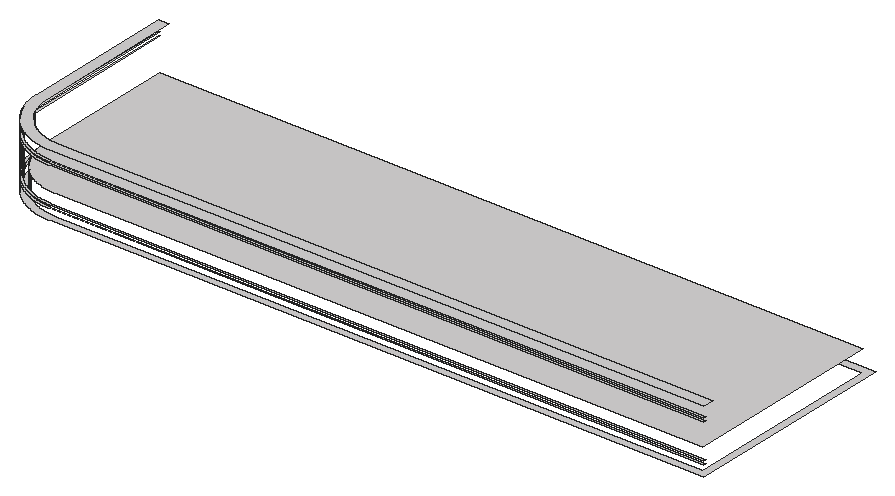
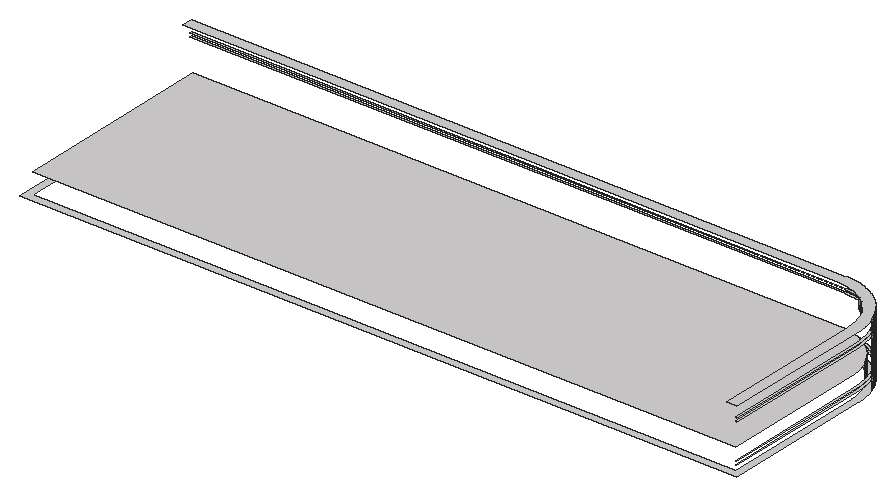
# SketchUp Ruby script. Lengths in inches.
U = 1.inch
M = Sketchup.active_model
def pt(a) = Geom::Point3d.new(a.map { |v| v * U })
def face(e, loops, mat)
  f = e.add_face(loops[0].map { |a| pt(a) })
  loops[1..].each { |l| e.add_face(l.map { |a| pt(a) }).erase! }
  f.material = f.back_material = mat if mat
  f
end
# faces: each face lists its corners as indices into pts; further lists are holes
def faces(e, pts, list, mat = nil) = list.each { |f| face(e, (f[0].is_a?(Array) ? f : [f]).map { |l| l.map { |i| pts[i] } }, mat) }
# xy, xz, yz: faces in a plane at the given z, y or x. An outline is a flat list of corners, or four numbers for a rectangle; further outlines are holes
def ring(l) = l.size == 4 ? [[l[0], l[1]], [l[2], l[1]], [l[2], l[3]], [l[0], l[3]]] : l.each_slice(2).to_a
def flat(e, list, mat, &to3) = list.each { |f| face(e, (f[0].is_a?(Array) ? f : [f]).map { |l| ring(l).map { |u, v| to3.(u, v) } }, mat) }
def xy(e, z, list, mat = nil) = flat(e, list, mat) { |x, y| [x, y, z] }
def xz(e, y, list, mat = nil) = flat(e, list, mat) { |x, z| [x, y, z] }
def yz(e, x, list, mat = nil) = flat(e, list, mat) { |y, z| [x, y, z] }
def lines(e, pts, list) = list.each { |a, b| e.add_line(pt(pts[a]), pt(pts[b])) }
# prism: a flat outline (further loops are holes) pulled along v
def prism(e, loops, v, mat = nil)
  f = face(e, loops, mat); d = Geom::Vector3d.new(v.map { |x| x * U })
  f.pushpull(f.normal.samedirection?(d) ? d.length : -d.length)
end
def box(e, o, s, mat = nil) = prism(e, [[o, [o[0] + s[0], o[1], o[2]], [o[0] + s[0], o[1] + s[1], o[2]], [o[0], o[1] + s[1], o[2]]]], [0, 0, s[2]], mat)
def at(x, y, z, deg = 0) = Geom::Transformation.translation(pt([x, y, z])) * Geom::Transformation.rotation(ORIGIN, Z_AXIS, deg.degrees)
def axes(o, x, y, z) = Geom::Transformation.new([*x, 0, *y, 0, *z, 0, *pt(o).to_a, 1])
def part(name) = M.definitions.add(name)
# library, detail: a bought-in or finely detailed component or shape, given as its bounding box
def library(name, o, s) = part(name).tap { |d| box(d.entities, o, s) }
def detail(e, o, s) = box(e.add_group.entities, o, s)
def put(e, d, t, mat = nil) = e.add_instance(d, t).tap { |i| i.material = mat if mat }
def group(e, t, mat = nil) = e.add_group.tap { |g| g.transformation = t; g.material = mat if mat }.entities
root = M.entities
M.materials.add("[Quartz Light Brown]").color = [215, 212, 212]
xy(root,243,[[[17.76,205,17.53,205.01,17.29,205.01,17.06,205.02,16.82,205.04,16.59,205.06,16.35,205.08,16.12,205.1,15.88,205.125,15.65,205.15,15.42,205.1875,15.18,205.22,14.72,205.3,14.49,205.35,14.26,205.39,14.03,205.44,13.8,205.5,13.57,205.55,13.34,205.61,13.11,205.68,12.89,205.74,12.66,205.81,12.4375,205.88,12.21,205.96,11.99,206.03,11.77,206.11,11.55,206.2,11.33,206.28,10.89,206.46,10.68,206.56,10.46,206.65,10.25,206.75,10.04,206.86,9.83,206.96,9.41,207.18,9.2,207.3,9,207.41,8.6,207.65,8.39,207.78,8.2,207.9,8,208.03,7.8,208.17,7.61,208.3,7.42,208.4375,7.23,208.58,7.04,208.72,6.86,208.86,6.67,209.01,6.49,209.16,6.31,209.3125,6.13,209.47,5.96,209.625,5.78,209.78,5.61,209.94,5.44,210.11,5.27,210.27,5.11,210.44,4.94,210.61,4.78,210.78,4.625,210.96,4.47,211.13,4.3125,211.31,4.16,211.49,4.01,211.67,3.86,211.86,3.72,212.04,3.58,212.23,3.4375,212.42,3.3,212.61,3.17,212.8,3.03,213,2.9,213.2,2.78,213.39,2.65,213.6,2.41,214,2.3,214.2,2.18,214.41,1.96,214.83,1.86,215.04,1.75,215.25,1.65,215.46,1.56,215.68,1.46,215.89,1.28,216.33,1.2,216.55,1.11,216.77,1.03,216.99,0.96,217.21,0.88,217.4375,0.81,217.66,0.74,217.89,0.68,218.11,0.61,218.34,0.55,218.57,0.5,218.8,0.44,219.03,0.39,219.26,0.35,219.49,0.3,219.72,0.22,220.18,0.1875,220.42,0.15,220.65,0.125,220.88,0.1,221.12,0.08,221.35,0.06,221.59,0.04,221.82,0.02,222.06,0.01,222.29,0.01,222.53,0,222.76,0,266,204,266,204,205],[17.79,207,202,207,202,264,2,264,2,222.79,2.01,222.58,2.01,222.37,2.03,221.95,2.05,221.74,2.07,221.54,2.11,221.12,2.17,220.7,2.2,220.5,2.23,220.29,2.27,220.08,2.31,219.88,2.35,219.67,2.39,219.47,2.44,219.26,2.49,219.0625,2.55,218.86,2.6,218.66,2.78,218.06,2.99,217.46,3.0625,217.27,3.14,217.07,3.22,216.88,3.3,216.68,3.38,216.49,3.65,215.92,3.74,215.74,3.84,215.55,3.9375,215.37,4.04,215.18,4.14,215,4.47,214.46,4.58,214.29,4.7,214.11,4.8125,213.9375,4.93,213.77,5.06,213.6,5.18,213.43,5.31,213.26,5.43,213.09,5.57,212.93,5.83,212.61,6.11,212.29,6.39,211.99,6.54,211.84,6.6875,211.6875,6.84,211.54,6.99,211.39,7.29,211.11,7.61,210.83,7.93,210.57,8.09,210.43,8.26,210.31,8.43,210.18,8.6,210.06,8.77,209.93,8.9375,209.8125,9.11,209.7,9.29,209.58,9.46,209.47,10,209.14,10.18,209.04,10.37,208.9375,10.55,208.84,10.74,208.74,10.92,208.65,11.49,208.38,11.68,208.3,11.88,208.22,12.07,208.14,12.27,208.0625,12.46,207.99,13.06,207.78,13.66,207.6,13.86,207.55,14.0625,207.49,14.26,207.44,14.47,207.39,14.67,207.35,14.88,207.31,15.08,207.27,15.29,207.23,15.5,207.2,15.7,207.17,16.12,207.11,16.54,207.07,16.74,207.05,16.95,207.03,17.37,207.01,17.58,207.01]]],"[Quartz Light Brown]")
xy(root,246,[[17.76,205,204,205,204,205.5,17.77,205.5,17.54,205.51,17.3125,205.51,17.08,205.52,16.86,205.54,16.625,205.55,16.4,205.57,16.17,205.6,15.94,205.62,15.72,205.65,15.49,205.68,15.26,205.72,15.04,205.75,14.8125,205.79,14.59,205.84,14.36,205.88,14.14,205.93,13.91,205.98,13.03,206.22,12.8125,206.29,12.59,206.36,12.16,206.5,11.94,206.58,11.73,206.66,11.52,206.75,11.3,206.83,10.88,207.01,10.67,207.11,10.47,207.2,10.26,207.3,10.06,207.41,9.85,207.51,9.25,207.84,9.05,207.96,8.86,208.08,8.66,208.2,8.47,208.32,7.71,208.84,6.99,209.4,6.81,209.55,6.63,209.69,6.29,209.99,5.95,210.31,5.79,210.46,5.46,210.79,5.31,210.95,4.99,211.29,4.69,211.63,4.55,211.81,4.4,211.99,3.84,212.71,3.32,213.47,3.2,213.66,3.08,213.86,2.96,214.05,2.84,214.25,2.51,214.85,2.41,215.06,2.3,215.26,2.2,215.47,2.11,215.67,2.01,215.88,1.83,216.3,1.75,216.52,1.66,216.73,1.58,216.94,1.5,217.16,1.36,217.59,1.29,217.8125,1.22,218.03,0.98,218.91,0.93,219.14,0.88,219.36,0.84,219.59,0.79,219.8125,0.75,220.04,0.72,220.26,0.68,220.49,0.65,220.72,0.62,220.94,0.6,221.17,0.57,221.4,0.55,221.625,0.54,221.86,0.52,222.08,0.51,222.3125,0.51,222.54,0.5,222.77,0.5,266,0,266,0,222.76,0.01,222.53,0.01,222.29,0.02,222.06,0.04,221.82,0.06,221.59,0.08,221.35,0.1,221.12,0.125,220.88,0.15,220.65,0.1875,220.42,0.22,220.18,0.3,219.72,0.35,219.49,0.39,219.26,0.44,219.03,0.5,218.8,0.55,218.57,0.61,218.34,0.68,218.11,0.74,217.89,0.81,217.66,0.88,217.4375,0.96,217.21,1.03,216.99,1.11,216.77,1.2,216.55,1.28,216.33,1.46,215.89,1.56,215.68,1.65,215.46,1.75,215.25,1.86,215.04,1.96,214.83,2.18,214.41,2.3,214.2,2.41,214,2.65,213.6,2.78,213.39,2.9,213.2,3.03,213,3.17,212.8,3.3,212.61,3.4375,212.42,3.58,212.23,3.72,212.04,3.86,211.86,4.01,211.67,4.16,211.49,4.3125,211.31,4.47,211.13,4.625,210.96,4.78,210.78,4.94,210.61,5.11,210.44,5.27,210.27,5.44,210.11,5.61,209.94,5.78,209.78,5.96,209.625,6.13,209.47,6.31,209.3125,6.49,209.16,6.67,209.01,6.86,208.86,7.04,208.72,7.23,208.58,7.42,208.4375,7.61,208.3,7.8,208.17,8,208.03,8.2,207.9,8.39,207.78,8.6,207.65,9,207.41,9.2,207.3,9.41,207.18,9.83,206.96,10.04,206.86,10.25,206.75,10.46,206.65,10.68,206.56,10.89,206.46,11.33,206.28,11.55,206.2,11.77,206.11,11.99,206.03,12.21,205.96,12.4375,205.88,12.66,205.81,12.89,205.74,13.11,205.68,13.34,205.61,13.57,205.55,13.8,205.5,14.03,205.44,14.26,205.39,14.49,205.35,14.72,205.3,15.18,205.22,15.42,205.1875,15.65,205.15,15.88,205.125,16.12,205.1,16.35,205.08,16.59,205.06,16.82,205.04,17.06,205.02,17.29,205.01,17.53,205.01]],"[Quartz Light Brown]")
xy(root,247,[[17.76,205,17.53,205.01,17.29,205.01,17.06,205.02,16.82,205.04,16.59,205.06,16.35,205.08,16.12,205.1,15.88,205.125,15.65,205.15,15.42,205.1875,15.18,205.22,14.72,205.3,14.49,205.35,14.26,205.39,14.03,205.44,13.8,205.5,13.57,205.55,13.34,205.61,13.11,205.68,12.89,205.74,12.66,205.81,12.4375,205.88,12.21,205.96,11.99,206.03,11.77,206.11,11.55,206.2,11.33,206.28,10.89,206.46,10.68,206.56,10.46,206.65,10.25,206.75,10.04,206.86,9.83,206.96,9.41,207.18,9.2,207.3,9,207.41,8.6,207.65,8.39,207.78,8.2,207.9,8,208.03,7.8,208.17,7.61,208.3,7.42,208.4375,7.23,208.58,7.04,208.72,6.86,208.86,6.67,209.01,6.49,209.16,6.31,209.3125,6.13,209.47,5.96,209.625,5.78,209.78,5.61,209.94,5.44,210.11,5.27,210.27,5.11,210.44,4.94,210.61,4.78,210.78,4.625,210.96,4.47,211.13,4.3125,211.31,4.16,211.49,4.01,211.67,3.86,211.86,3.72,212.04,3.58,212.23,3.4375,212.42,3.3,212.61,3.17,212.8,3.03,213,2.9,213.2,2.78,213.39,2.65,213.6,2.41,214,2.3,214.2,2.18,214.41,1.96,214.83,1.86,215.04,1.75,215.25,1.65,215.46,1.56,215.68,1.46,215.89,1.28,216.33,1.2,216.55,1.11,216.77,1.03,216.99,0.96,217.21,0.88,217.4375,0.81,217.66,0.74,217.89,0.68,218.11,0.61,218.34,0.55,218.57,0.5,218.8,0.44,219.03,0.39,219.26,0.35,219.49,0.3,219.72,0.22,220.18,0.1875,220.42,0.15,220.65,0.125,220.88,0.1,221.12,0.08,221.35,0.06,221.59,0.04,221.82,0.02,222.06,0.01,222.29,0.01,222.53,0,222.76,0,266,0.5,266,0.5,222.77,0.51,222.54,0.51,222.3125,0.52,222.08,0.54,221.86,0.55,221.625,0.57,221.4,0.6,221.17,0.62,220.94,0.65,220.72,0.68,220.49,0.72,220.26,0.75,220.04,0.79,219.8125,0.84,219.59,0.88,219.36,0.93,219.14,0.98,218.91,1.22,218.03,1.29,217.8125,1.36,217.59,1.5,217.16,1.58,216.94,1.66,216.73,1.75,216.52,1.83,216.3,2.01,215.88,2.11,215.67,2.2,215.47,2.3,215.26,2.41,215.06,2.51,214.85,2.84,214.25,2.96,214.05,3.08,213.86,3.2,213.66,3.32,213.47,3.84,212.71,4.4,211.99,4.55,211.81,4.69,211.63,4.99,211.29,5.31,210.95,5.46,210.79,5.79,210.46,5.95,210.31,6.29,209.99,6.63,209.69,6.81,209.55,6.99,209.4,7.71,208.84,8.47,208.32,8.66,208.2,8.86,208.08,9.05,207.96,9.25,207.84,9.85,207.51,10.06,207.41,10.26,207.3,10.47,207.2,10.67,207.11,10.88,207.01,11.3,206.83,11.52,206.75,11.73,206.66,11.94,206.58,12.16,206.5,12.59,206.36,12.8125,206.29,13.03,206.22,13.91,205.98,14.14,205.93,14.36,205.88,14.59,205.84,14.8125,205.79,15.04,205.75,15.26,205.72,15.49,205.68,15.72,205.65,15.94,205.62,16.17,205.6,16.4,205.57,16.625,205.55,16.86,205.54,17.08,205.52,17.3125,205.51,17.54,205.51,17.77,205.5,204,205.5,204,205]],"[Quartz Light Brown]")
xy(root,249,[[17.79,207,17.58,207.01,17.37,207.01,16.95,207.03,16.74,207.05,16.54,207.07,16.12,207.11,15.7,207.17,15.5,207.2,15.29,207.23,15.08,207.27,14.88,207.31,14.67,207.35,14.47,207.39,14.26,207.44,14.0625,207.49,13.86,207.55,13.66,207.6,13.06,207.78,12.46,207.99,12.27,208.0625,12.07,208.14,11.88,208.22,11.68,208.3,11.49,208.38,10.92,208.65,10.74,208.74,10.55,208.84,10.37,208.9375,10.18,209.04,10,209.14,9.46,209.47,9.29,209.58,9.11,209.7,8.9375,209.8125,8.77,209.93,8.6,210.06,8.43,210.18,8.26,210.31,8.09,210.43,7.93,210.57,7.61,210.83,7.29,211.11,6.99,211.39,6.84,211.54,6.6875,211.6875,6.54,211.84,6.39,211.99,6.11,212.29,5.83,212.61,5.57,212.93,5.43,213.09,5.31,213.26,5.18,213.43,5.06,213.6,4.93,213.77,4.8125,213.9375,4.7,214.11,4.58,214.29,4.47,214.46,4.14,215,4.04,215.18,3.9375,215.37,3.84,215.55,3.74,215.74,3.65,215.92,3.38,216.49,3.3,216.68,3.22,216.88,3.14,217.07,3.0625,217.27,2.99,217.46,2.78,218.06,2.6,218.66,2.55,218.86,2.49,219.0625,2.44,219.26,2.39,219.47,2.35,219.67,2.31,219.88,2.27,220.08,2.23,220.29,2.2,220.5,2.17,220.7,2.11,221.12,2.07,221.54,2.05,221.74,2.03,221.95,2.01,222.37,2.01,222.58,2,222.79,2,264,202,264,202,207]],"[Quartz Light Brown]")
xy(root,257,[[17.76,205,204,205,204,205.5,17.77,205.5,17.54,205.51,17.3125,205.51,17.08,205.52,16.86,205.54,16.625,205.55,16.4,205.57,16.17,205.6,15.94,205.62,15.72,205.65,15.49,205.68,15.26,205.72,15.04,205.75,14.8125,205.79,14.59,205.84,14.36,205.88,14.14,205.93,13.91,205.98,13.03,206.22,12.8125,206.29,12.59,206.36,12.16,206.5,11.94,206.58,11.73,206.66,11.52,206.75,11.3,206.83,10.88,207.01,10.67,207.11,10.47,207.2,10.26,207.3,10.06,207.41,9.85,207.51,9.25,207.84,9.05,207.96,8.86,208.08,8.66,208.2,8.47,208.32,7.71,208.84,6.99,209.4,6.81,209.55,6.63,209.69,6.29,209.99,5.95,210.31,5.79,210.46,5.46,210.79,5.31,210.95,4.99,211.29,4.69,211.63,4.55,211.81,4.4,211.99,3.84,212.71,3.32,213.47,3.2,213.66,3.08,213.86,2.96,214.05,2.84,214.25,2.51,214.85,2.41,215.06,2.3,215.26,2.2,215.47,2.11,215.67,2.01,215.88,1.83,216.3,1.75,216.52,1.66,216.73,1.58,216.94,1.5,217.16,1.36,217.59,1.29,217.8125,1.22,218.03,0.98,218.91,0.93,219.14,0.88,219.36,0.84,219.59,0.79,219.8125,0.75,220.04,0.72,220.26,0.68,220.49,0.65,220.72,0.62,220.94,0.6,221.17,0.57,221.4,0.55,221.625,0.54,221.86,0.52,222.08,0.51,222.3125,0.51,222.54,0.5,222.77,0.5,266,0,266,0,222.76,0.01,222.53,0.01,222.29,0.02,222.06,0.04,221.82,0.06,221.59,0.08,221.35,0.1,221.12,0.125,220.88,0.15,220.65,0.1875,220.42,0.22,220.18,0.3,219.72,0.35,219.49,0.39,219.26,0.44,219.03,0.5,218.8,0.55,218.57,0.61,218.34,0.68,218.11,0.74,217.89,0.81,217.66,0.88,217.4375,0.96,217.21,1.03,216.99,1.11,216.77,1.2,216.55,1.28,216.33,1.46,215.89,1.56,215.68,1.65,215.46,1.75,215.25,1.86,215.04,1.96,214.83,2.18,214.41,2.3,214.2,2.41,214,2.65,213.6,2.78,213.39,2.9,213.2,3.03,213,3.17,212.8,3.3,212.61,3.4375,212.42,3.58,212.23,3.72,212.04,3.86,211.86,4.01,211.67,4.16,211.49,4.3125,211.31,4.47,211.13,4.625,210.96,4.78,210.78,4.94,210.61,5.11,210.44,5.27,210.27,5.44,210.11,5.61,209.94,5.78,209.78,5.96,209.625,6.13,209.47,6.31,209.3125,6.49,209.16,6.67,209.01,6.86,208.86,7.04,208.72,7.23,208.58,7.42,208.4375,7.61,208.3,7.8,208.17,8,208.03,8.2,207.9,8.39,207.78,8.6,207.65,9,207.41,9.2,207.3,9.41,207.18,9.83,206.96,10.04,206.86,10.25,206.75,10.46,206.65,10.68,206.56,10.89,206.46,11.33,206.28,11.55,206.2,11.77,206.11,11.99,206.03,12.21,205.96,12.4375,205.88,12.66,205.81,12.89,205.74,13.11,205.68,13.34,205.61,13.57,205.55,13.8,205.5,14.03,205.44,14.26,205.39,14.49,205.35,14.72,205.3,15.18,205.22,15.42,205.1875,15.65,205.15,15.88,205.125,16.12,205.1,16.35,205.08,16.59,205.06,16.82,205.04,17.06,205.02,17.29,205.01,17.53,205.01]],"[Quartz Light Brown]")
xy(root,258,[[17.76,205,17.53,205.01,17.29,205.01,17.06,205.02,16.82,205.04,16.59,205.06,16.35,205.08,16.12,205.1,15.88,205.125,15.65,205.15,15.42,205.1875,15.18,205.22,14.72,205.3,14.49,205.35,14.26,205.39,14.03,205.44,13.8,205.5,13.57,205.55,13.34,205.61,13.11,205.68,12.89,205.74,12.66,205.81,12.4375,205.88,12.21,205.96,11.99,206.03,11.77,206.11,11.55,206.2,11.33,206.28,10.89,206.46,10.68,206.56,10.46,206.65,10.25,206.75,10.04,206.86,9.83,206.96,9.41,207.18,9.2,207.3,9,207.41,8.6,207.65,8.39,207.78,8.2,207.9,8,208.03,7.8,208.17,7.61,208.3,7.42,208.4375,7.23,208.58,7.04,208.72,6.86,208.86,6.67,209.01,6.49,209.16,6.31,209.3125,6.13,209.47,5.96,209.625,5.78,209.78,5.61,209.94,5.44,210.11,5.27,210.27,5.11,210.44,4.94,210.61,4.78,210.78,4.625,210.96,4.47,211.13,4.3125,211.31,4.16,211.49,4.01,211.67,3.86,211.86,3.72,212.04,3.58,212.23,3.4375,212.42,3.3,212.61,3.17,212.8,3.03,213,2.9,213.2,2.78,213.39,2.65,213.6,2.41,214,2.3,214.2,2.18,214.41,1.96,214.83,1.86,215.04,1.75,215.25,1.65,215.46,1.56,215.68,1.46,215.89,1.28,216.33,1.2,216.55,1.11,216.77,1.03,216.99,0.96,217.21,0.88,217.4375,0.81,217.66,0.74,217.89,0.68,218.11,0.61,218.34,0.55,218.57,0.5,218.8,0.44,219.03,0.39,219.26,0.35,219.49,0.3,219.72,0.22,220.18,0.1875,220.42,0.15,220.65,0.125,220.88,0.1,221.12,0.08,221.35,0.06,221.59,0.04,221.82,0.02,222.06,0.01,222.29,0.01,222.53,0,222.76,0,266,0.5,266,0.5,222.77,0.51,222.54,0.51,222.3125,0.52,222.08,0.54,221.86,0.55,221.625,0.57,221.4,0.6,221.17,0.62,220.94,0.65,220.72,0.68,220.49,0.72,220.26,0.75,220.04,0.79,219.8125,0.84,219.59,0.88,219.36,0.93,219.14,0.98,218.91,1.22,218.03,1.29,217.8125,1.36,217.59,1.5,217.16,1.58,216.94,1.66,216.73,1.75,216.52,1.83,216.3,2.01,215.88,2.11,215.67,2.2,215.47,2.3,215.26,2.41,215.06,2.51,214.85,2.84,214.25,2.96,214.05,3.08,213.86,3.2,213.66,3.32,213.47,3.84,212.71,4.4,211.99,4.55,211.81,4.69,211.63,4.99,211.29,5.31,210.95,5.46,210.79,5.79,210.46,5.95,210.31,6.29,209.99,6.63,209.69,6.81,209.55,6.99,209.4,7.71,208.84,8.47,208.32,8.66,208.2,8.86,208.08,9.05,207.96,9.25,207.84,9.85,207.51,10.06,207.41,10.26,207.3,10.47,207.2,10.67,207.11,10.88,207.01,11.3,206.83,11.52,206.75,11.73,206.66,11.94,206.58,12.16,206.5,12.59,206.36,12.8125,206.29,13.03,206.22,13.91,205.98,14.14,205.93,14.36,205.88,14.59,205.84,14.8125,205.79,15.04,205.75,15.26,205.72,15.49,205.68,15.72,205.65,15.94,205.62,16.17,205.6,16.4,205.57,16.625,205.55,16.86,205.54,17.08,205.52,17.3125,205.51,17.54,205.51,17.77,205.5,204,205.5,204,205]],"[Quartz Light Brown]")
xy(root,261,[[17.76,205,204,205,204,208,17.8,208,17.61,208.01,17.41,208.01,17.21,208.02,17.02,208.03,16.82,208.05,16.63,208.0625,16.43,208.08,16.24,208.1,16.04,208.13,15.85,208.16,15.65,208.18,15.46,208.22,15.27,208.25,15.07,208.29,14.5,208.41,14.12,208.51,13.93,208.5625,13.74,208.62,13.55,208.67,13.36,208.73,13.18,208.8,12.99,208.86,12.81,208.93,12.44,209.07,12.26,209.14,11.54,209.46,11.37,209.55,11.19,209.63,11.02,209.73,10.84,209.82,10.67,209.91,10.16,210.21,10,210.3125,9.83,210.42,9.67,210.53,9.5,210.64,9.18,210.86,9.03,210.98,8.71,211.22,8.56,211.34,8.41,211.47,8.26,211.59,7.96,211.85,7.82,211.99,7.67,212.12,7.53,212.26,7.39,212.39,7.26,212.53,7.12,212.67,6.99,212.82,6.85,212.96,6.59,213.26,6.47,213.41,6.34,213.56,6.22,213.71,5.98,214.03,5.86,214.18,5.64,214.5,5.53,214.67,5.42,214.83,5.3125,215,5.21,215.16,4.91,215.67,4.82,215.84,4.73,216.02,4.63,216.19,4.55,216.37,4.46,216.54,4.14,217.26,4.07,217.44,3.93,217.81,3.86,217.99,3.8,218.18,3.73,218.36,3.67,218.55,3.62,218.74,3.5625,218.93,3.51,219.12,3.41,219.5,3.29,220.07,3.25,220.27,3.22,220.46,3.18,220.65,3.16,220.85,3.13,221.04,3.1,221.24,3.08,221.43,3.0625,221.63,3.05,221.82,3.03,222.02,3.02,222.21,3.01,222.41,3.01,222.61,3,222.8,3,266,0,266,0,222.76,0.01,222.53,0.01,222.29,0.02,222.06,0.04,221.82,0.06,221.59,0.08,221.35,0.1,221.12,0.125,220.88,0.15,220.65,0.1875,220.42,0.22,220.18,0.3,219.72,0.35,219.49,0.39,219.26,0.44,219.03,0.5,218.8,0.55,218.57,0.61,218.34,0.68,218.11,0.74,217.89,0.81,217.66,0.88,217.4375,0.96,217.21,1.03,216.99,1.11,216.77,1.2,216.55,1.28,216.33,1.46,215.89,1.56,215.68,1.65,215.46,1.75,215.25,1.86,215.04,1.96,214.83,2.18,214.41,2.3,214.2,2.41,214,2.65,213.6,2.78,213.39,2.9,213.2,3.03,213,3.17,212.8,3.3,212.61,3.4375,212.42,3.58,212.23,3.72,212.04,3.86,211.86,4.01,211.67,4.16,211.49,4.3125,211.31,4.47,211.13,4.625,210.96,4.78,210.78,4.94,210.61,5.11,210.44,5.27,210.27,5.44,210.11,5.61,209.94,5.78,209.78,5.96,209.625,6.13,209.47,6.31,209.3125,6.49,209.16,6.67,209.01,6.86,208.86,7.04,208.72,7.23,208.58,7.42,208.4375,7.61,208.3,7.8,208.17,8,208.03,8.2,207.9,8.39,207.78,8.6,207.65,9,207.41,9.2,207.3,9.41,207.18,9.83,206.96,10.04,206.86,10.25,206.75,10.46,206.65,10.68,206.56,10.89,206.46,11.33,206.28,11.55,206.2,11.77,206.11,11.99,206.03,12.21,205.96,12.4375,205.88,12.66,205.81,12.89,205.74,13.11,205.68,13.34,205.61,13.57,205.55,13.8,205.5,14.03,205.44,14.26,205.39,14.49,205.35,14.72,205.3,15.18,205.22,15.42,205.1875,15.65,205.15,15.88,205.125,16.12,205.1,16.35,205.08,16.59,205.06,16.82,205.04,17.06,205.02,17.29,205.01,17.53,205.01]],"[Quartz Light Brown]")
p = [[5.11,210.44,246],[5.11,210.44,243],[5.27,210.27,243],[5.27,210.27,246],[8.09,210.43,249],[8.26,210.31,249],
  [8.26,210.31,243],[8.09,210.43,243],[4.94,210.61,246],[4.94,210.61,243],[7.93,210.57,249],[7.93,210.57,243],
  [4.78,210.78,246],[4.78,210.78,243],[7.77,210.7,249],[7.77,210.7,243],[7.61,210.83,249],[7.61,210.83,243],
  [4.625,210.96,246],[4.625,210.96,243],[7.45,210.97,249],[7.45,210.97,243],[4.47,211.13,246],[4.47,211.13,243],
  [7.29,211.11,249],[7.29,211.11,243],[4.3125,211.31,246],[4.3125,211.31,243],[7.14,211.25,249],[7.14,211.25,243],
  [4.16,211.49,246],[4.16,211.49,243],[6.99,211.39,249],[6.99,211.39,243],[6.84,211.54,249],[6.84,211.54,243],
  [4.01,211.67,246],[4.01,211.67,243],[6.6875,211.6875,249],[6.6875,211.6875,243],[3.86,211.86,246],[3.86,211.86,243],
  [6.54,211.84,249],[6.54,211.84,243],[6.39,211.99,249],[6.39,211.99,243],[3.72,212.04,246],[3.72,212.04,243],
  [3.58,212.23,246],[3.58,212.23,243],[6.25,212.14,249],[6.25,212.14,243],[6.11,212.29,249],[6.11,212.29,243],
  [3.4375,212.42,246],[3.4375,212.42,243],[5.97,212.45,249],[5.97,212.45,243],[3.3,212.61,246],[3.3,212.61,243],
  [5.83,212.61,249],[5.83,212.61,243],[3.17,212.8,246],[3.17,212.8,243],[5.7,212.77,249],[5.7,212.77,243],
  [3.03,213,246],[3.03,213,243],[5.57,212.93,249],[5.57,212.93,243],[5.43,213.09,249],[5.43,213.09,243],
  [2.9,213.2,246],[2.9,213.2,243],[5.31,213.26,249],[5.31,213.26,243],[2.78,213.39,246],[2.78,213.39,243],
  [5.18,213.43,249],[5.18,213.43,243],[2.65,213.6,246],[2.65,213.6,243],[5.06,213.6,249],[5.06,213.6,243],
  [2.53,213.8,246],[2.53,213.8,243],[4.93,213.77,249],[4.93,213.77,243],[2.41,214,246],[2.41,214,243],
  [4.8125,213.9375,249],[4.8125,213.9375,243],[4.7,214.11,249],[4.7,214.11,243],[2.3,214.2,246],[2.3,214.2,243],
  [4.58,214.29,249],[4.58,214.29,243],[2.18,214.41,246],[2.18,214.41,243],[4.47,214.46,249],[4.47,214.46,243],
  [2.07,214.62,246],[2.07,214.62,243],[4.36,214.64,249],[4.36,214.64,243],[1.96,214.83,246],[1.96,214.83,243],
  [4.25,214.82,249],[4.25,214.82,243],[1.86,215.04,246],[1.86,215.04,243],[4.14,215,249],[4.14,215,243],
  [1.75,215.25,246],[1.75,215.25,243],[4.04,215.18,249],[4.04,215.18,243],[3.9375,215.37,249],[3.9375,215.37,243],
  [1.65,215.46,246],[1.65,215.46,243],[3.84,215.55,249],[3.84,215.55,243],[1.56,215.68,246],[1.56,215.68,243],
  [3.74,215.74,249],[3.74,215.74,243],[1.46,215.89,246],[1.46,215.89,243],[3.65,215.92,249],[3.65,215.92,243],
  [1.37,216.11,246],[1.37,216.11,243],[3.56,216.11,249],[3.56,216.11,243],[1.28,216.33,246],[1.28,216.33,243],
  [3.47,216.3,249],[3.47,216.3,243],[5.79,210.46,247],[5.79,210.46,246],[5.95,210.31,246],[5.95,210.31,247],
  [5.625,210.625,247],[5.625,210.625,246],[5.46,210.79,247],[5.46,210.79,246],[5.31,210.95,247],[5.31,210.95,246],
  [5.15,211.12,247],[5.15,211.12,246],[4.99,211.29,247],[4.99,211.29,246],[4.84,211.46,247],[4.84,211.46,246],
  [4.69,211.63,247],[4.69,211.63,246],[4.55,211.81,247],[4.55,211.81,246],[4.4,211.99,247],[4.4,211.99,246],
  [4.26,212.17,247],[4.26,212.17,246],[4.12,212.35,247],[4.12,212.35,246],[3.98,212.53,247],[3.98,212.53,246],
  [3.84,212.71,247],[3.84,212.71,246],[3.71,212.9,247],[3.71,212.9,246],[3.58,213.09,247],[3.58,213.09,246],
  [3.45,213.28,247],[3.45,213.28,246],[3.32,213.47,247],[3.32,213.47,246],[3.2,213.66,247],[3.2,213.66,246],
  [3.08,213.86,247],[3.08,213.86,246],[2.96,214.05,247],[2.96,214.05,246],[2.84,214.25,247],[2.84,214.25,246],
  [2.73,214.45,247],[2.73,214.45,246],[2.62,214.65,247],[2.62,214.65,246],[2.51,214.85,247],[2.51,214.85,246],
  [2.41,215.06,247],[2.41,215.06,246],[2.3,215.26,247],[2.3,215.26,246],[2.2,215.47,247],[2.2,215.47,246],
  [2.11,215.67,247],[2.11,215.67,246],[2.01,215.88,247],[2.01,215.88,246],[1.92,216.09,247],[1.92,216.09,246],
  [1.83,216.3,247],[1.83,216.3,246],[5.11,210.44,257],[5.11,210.44,247],[5.27,210.27,247],[5.27,210.27,257],
  [4.94,210.61,257],[4.94,210.61,247],[4.78,210.78,257],[4.78,210.78,247],[4.625,210.96,257],[4.625,210.96,247],
  [4.47,211.13,257],[4.47,211.13,247],[4.3125,211.31,257],[4.3125,211.31,247],[4.16,211.49,257],[4.16,211.49,247],
  [4.01,211.67,257],[4.01,211.67,247],[3.86,211.86,257],[3.86,211.86,247],[3.72,212.04,257],[3.72,212.04,247],
  [3.58,212.23,257],[3.58,212.23,247],[3.4375,212.42,257],[3.4375,212.42,247],[3.3,212.61,257],[3.3,212.61,247],
  [3.17,212.8,257],[3.17,212.8,247],[3.03,213,257],[3.03,213,247],[2.9,213.2,257],[2.9,213.2,247],
  [2.78,213.39,257],[2.78,213.39,247],[2.65,213.6,257],[2.65,213.6,247],[2.53,213.8,257],[2.53,213.8,247],
  [2.41,214,257],[2.41,214,247],[2.3,214.2,257],[2.3,214.2,247],[2.18,214.41,257],[2.18,214.41,247],
  [2.07,214.62,257],[2.07,214.62,247],[1.96,214.83,257],[1.96,214.83,247],[1.86,215.04,257],[1.86,215.04,247],
  [1.75,215.25,257],[1.75,215.25,247],[1.65,215.46,257],[1.65,215.46,247],[1.56,215.68,257],[1.56,215.68,247],
  [1.46,215.89,257],[1.46,215.89,247],[1.37,216.11,257],[1.37,216.11,247],[1.28,216.33,257],[1.28,216.33,247],
  [5.79,210.46,258],[5.79,210.46,257],[5.95,210.31,257],[5.95,210.31,258],[5.625,210.625,258],[5.625,210.625,257],
  [5.46,210.79,258],[5.46,210.79,257],[5.31,210.95,258],[5.31,210.95,257],[5.15,211.12,258],[5.15,211.12,257],
  [4.99,211.29,258],[4.99,211.29,257],[4.84,211.46,258],[4.84,211.46,257],[4.69,211.63,258],[4.69,211.63,257],
  [4.55,211.81,258],[4.55,211.81,257],[4.4,211.99,258],[4.4,211.99,257],[4.26,212.17,258],[4.26,212.17,257],
  [4.12,212.35,258],[4.12,212.35,257],[3.98,212.53,258],[3.98,212.53,257],[3.84,212.71,258],[3.84,212.71,257],
  [3.71,212.9,258],[3.71,212.9,257],[3.58,213.09,258],[3.58,213.09,257],[3.45,213.28,258],[3.45,213.28,257],
  [3.32,213.47,258],[3.32,213.47,257],[3.2,213.66,258],[3.2,213.66,257],[3.08,213.86,258],[3.08,213.86,257],
  [2.96,214.05,258],[2.96,214.05,257],[2.84,214.25,258],[2.84,214.25,257],[2.73,214.45,258],[2.73,214.45,257],
  [2.62,214.65,258],[2.62,214.65,257],[2.51,214.85,258],[2.51,214.85,257],[2.41,215.06,258],[2.41,215.06,257],
  [2.3,215.26,258],[2.3,215.26,257],[2.2,215.47,258],[2.2,215.47,257],[2.11,215.67,258],[2.11,215.67,257],
  [2.01,215.88,258],[2.01,215.88,257],[1.92,216.09,258],[1.92,216.09,257],[1.83,216.3,258],[1.83,216.3,257],
  [5.27,210.27,258],[5.27,210.27,261],[5.11,210.44,261],[5.11,210.44,258],[10,210.3125,258],[9.83,210.42,258],
  [9.83,210.42,261],[10,210.3125,261],[4.94,210.61,261],[4.94,210.61,258],[9.67,210.53,258],[9.67,210.53,261],
  [9.5,210.64,258],[9.5,210.64,261],[4.78,210.78,261],[4.78,210.78,258],[9.34,210.75,258],[9.34,210.75,261],
  [4.625,210.96,261],[4.625,210.96,258],[9.18,210.86,258],[9.18,210.86,261],[9.03,210.98,258],[9.03,210.98,261],
  [4.47,211.13,261],[4.47,211.13,258],[8.87,211.1,258],[8.87,211.1,261],[4.3125,211.31,261],[4.3125,211.31,258],
  [8.71,211.22,258],[8.71,211.22,261],[8.56,211.34,258],[8.56,211.34,261],[4.16,211.49,261],[4.16,211.49,258],
  [8.41,211.47,258],[8.41,211.47,261],[4.01,211.67,261],[4.01,211.67,258],[8.26,211.59,258],[8.26,211.59,261],
  [8.11,211.72,258],[8.11,211.72,261],[3.86,211.86,261],[3.86,211.86,258],[7.96,211.85,258],[7.96,211.85,261],
  [3.72,212.04,261],[3.72,212.04,258],[7.82,211.99,258],[7.82,211.99,261],[3.58,212.23,261],[3.58,212.23,258],
  [7.67,212.12,258],[7.67,212.12,261],[7.53,212.26,258],[7.53,212.26,261],[3.4375,212.42,261],[3.4375,212.42,258],
  [7.39,212.39,258],[7.39,212.39,261],[3.3,212.61,261],[3.3,212.61,258],[7.26,212.53,258],[7.26,212.53,261],
  [7.12,212.67,258],[7.12,212.67,261],[3.17,212.8,261],[3.17,212.8,258],[6.99,212.82,258],[6.99,212.82,261],
  [3.03,213,261],[3.03,213,258],[6.85,212.96,258],[6.85,212.96,261],[2.9,213.2,261],[2.9,213.2,258],
  [6.72,213.11,258],[6.72,213.11,261],[6.59,213.26,258],[6.59,213.26,261],[2.78,213.39,261],[2.78,213.39,258],
  [6.47,213.41,258],[6.47,213.41,261],[2.65,213.6,261],[2.65,213.6,258],[6.34,213.56,258],[6.34,213.56,261],
  [2.53,213.8,261],[2.53,213.8,258],[6.22,213.71,258],[6.22,213.71,261],[6.1,213.87,258],[6.1,213.87,261],
  [2.41,214,261],[2.41,214,258],[5.98,214.03,258],[5.98,214.03,261],[2.3,214.2,261],[2.3,214.2,258],
  [5.86,214.18,258],[5.86,214.18,261],[2.18,214.41,261],[2.18,214.41,258],[5.75,214.34,258],[5.75,214.34,261],
  [5.64,214.5,258],[5.64,214.5,261],[2.07,214.62,261],[2.07,214.62,258],[5.53,214.67,258],[5.53,214.67,261],
  [1.96,214.83,261],[1.96,214.83,258],[5.42,214.83,258],[5.42,214.83,261],[1.86,215.04,261],[1.86,215.04,258],
  [5.3125,215,258],[5.3125,215,261],[1.75,215.25,261],[1.75,215.25,258],[5.21,215.16,258],[5.21,215.16,261],
  [5.11,215.33,258],[5.11,215.33,261],[1.65,215.46,261],[1.65,215.46,258],[5.01,215.5,258],[5.01,215.5,261],
  [1.56,215.68,261],[1.56,215.68,258],[4.91,215.67,258],[4.91,215.67,261],[1.46,215.89,261],[1.46,215.89,258],
  [4.82,215.84,258],[4.82,215.84,261],[4.73,216.02,258],[4.73,216.02,261],[1.37,216.11,261],[1.37,216.11,258],
  [4.63,216.19,258],[4.63,216.19,261],[1.28,216.33,261],[1.28,216.33,258]]
faces(root,p,[[0,1,2,3],[4,5,6,7],[8,9,1,0],[10,4,7,11],[12,13,9,8],[14,10,11,15],[16,14,15,17],[18,19,13,12],
  [20,16,17,21],[22,23,19,18],[24,20,21,25],[26,27,23,22],[28,24,25,29],[30,31,27,26],[32,28,29,33],[34,32,33,35],
  [36,37,31,30],[38,34,35,39],[40,41,37,36],[42,38,39,43],[44,42,43,45],[46,47,41,40],[48,49,47,46],[50,44,45,51],
  [52,50,51,53],[54,55,49,48],[56,52,53,57],[58,59,55,54],[60,56,57,61],[62,63,59,58],[64,60,61,65],[66,67,63,62],
  [68,64,65,69],[70,68,69,71],[72,73,67,66],[74,70,71,75],[76,77,73,72],[78,74,75,79],[80,81,77,76],[82,78,79,83],
  [84,85,81,80],[86,82,83,87],[88,89,85,84],[90,86,87,91],[92,90,91,93],[94,95,89,88],[96,92,93,97],[98,99,95,94],
  [100,96,97,101],[102,103,99,98],[104,100,101,105],[106,107,103,102],[108,104,105,109],[110,111,107,106],[112,108,109,113],[114,115,111,110],
  [116,112,113,117],[118,116,117,119],[120,121,115,114],[122,118,119,123],[124,125,121,120],[126,122,123,127],[128,129,125,124],[130,126,127,131],
  [132,133,129,128],[134,130,131,135],[136,137,133,132],[138,134,135,139],[140,141,142,143],[144,145,141,140],[146,147,145,144],[148,149,147,146],
  [150,151,149,148],[152,153,151,150],[154,155,153,152],[156,157,155,154],[158,159,157,156],[160,161,159,158],[162,163,161,160],[164,165,163,162],
  [166,167,165,164],[168,169,167,166],[170,171,169,168],[172,173,171,170],[174,175,173,172],[176,177,175,174],[178,179,177,176],[180,181,179,178],
  [182,183,181,180],[184,185,183,182],[186,187,185,184],[188,189,187,186],[190,191,189,188],[192,193,191,190],[194,195,193,192],[196,197,195,194],
  [198,199,197,196],[200,201,199,198],[202,203,201,200],[204,205,203,202],[206,207,208,209],[210,211,207,206],[212,213,211,210],[214,215,213,212],
  [216,217,215,214],[218,219,217,216],[220,221,219,218],[222,223,221,220],[224,225,223,222],[226,227,225,224],[228,229,227,226],[230,231,229,228],
  [232,233,231,230],[234,235,233,232],[236,237,235,234],[238,239,237,236],[240,241,239,238],[242,243,241,240],[244,245,243,242],[246,247,245,244],
  [248,249,247,246],[250,251,249,248],[252,253,251,250],[254,255,253,252],[256,257,255,254],[258,259,257,256],[260,261,259,258],[262,263,261,260],
  [264,265,263,262],[266,267,265,264],[268,269,267,266],[270,271,272,273],[274,275,271,270],[276,277,275,274],[278,279,277,276],[280,281,279,278],
  [282,283,281,280],[284,285,283,282],[286,287,285,284],[288,289,287,286],[290,291,289,288],[292,293,291,290],[294,295,293,292],[296,297,295,294],
  [298,299,297,296],[300,301,299,298],[302,303,301,300],[304,305,303,302],[306,307,305,304],[308,309,307,306],[310,311,309,308],[312,313,311,310],
  [314,315,313,312],[316,317,315,314],[318,319,317,316],[320,321,319,318],[322,323,321,320],[324,325,323,322],[326,327,325,324],[328,329,327,326],
  [330,331,329,328],[332,333,331,330],[334,335,333,332],[336,337,338,339],[340,341,342,343],[339,338,344,345],[341,346,347,342],[346,348,349,347],
  [345,344,350,351],[348,352,353,349],[351,350,354,355],[352,356,357,353],[356,358,359,357],[355,354,360,361],[358,362,363,359],[361,360,364,365],
  [362,366,367,363],[366,368,369,367],[365,364,370,371],[368,372,373,369],[371,370,374,375],[372,376,377,373],[376,378,379,377],[375,374,380,381],
  [378,382,383,379],[381,380,384,385],[382,386,387,383],[385,384,388,389],[386,390,391,387],[390,392,393,391],[389,388,394,395],[392,396,397,393],
  [395,394,398,399],[396,400,401,397],[400,402,403,401],[399,398,404,405],[402,406,407,403],[405,404,408,409],[406,410,411,407],[409,408,412,413],
  [410,414,415,411],[414,416,417,415],[413,412,418,419],[416,420,421,417],[419,418,422,423],[420,424,425,421],[423,422,426,427],[424,428,429,425],
  [428,430,431,429],[427,426,432,433],[430,434,435,431],[433,432,436,437],[434,438,439,435],[437,436,440,441],[438,442,443,439],[442,444,445,443],
  [441,440,446,447],[444,448,449,445],[447,446,450,451],[448,452,453,449],[451,450,454,455],[452,456,457,453],[455,454,458,459],[456,460,461,457],
  [460,462,463,461],[459,458,464,465],[462,466,467,463],[465,464,468,469],[466,470,471,467],[469,468,472,473],[470,474,475,471],[474,476,477,475],
  [473,472,478,479],[476,480,481,477],[479,478,482,483]],"[Quartz Light Brown]")
